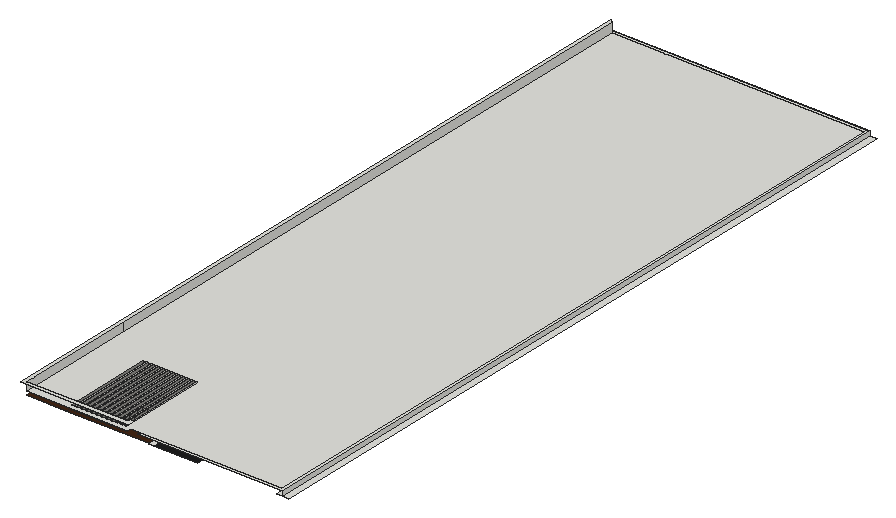
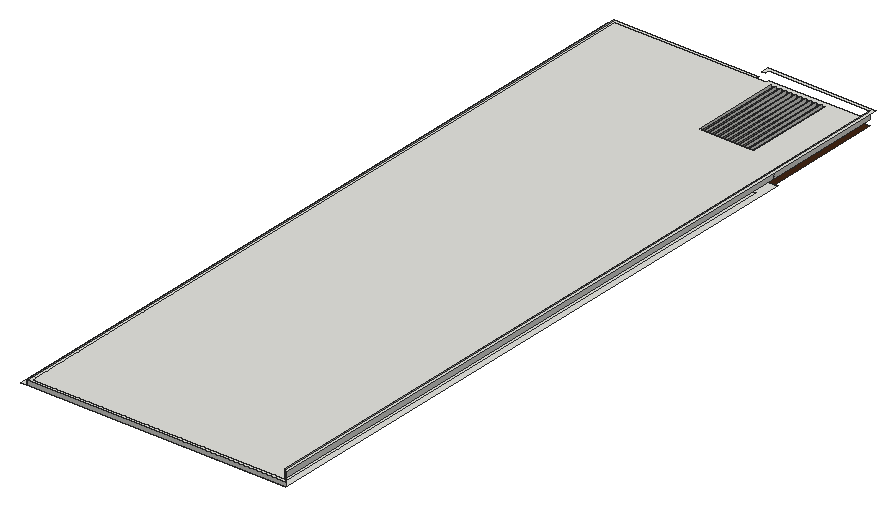
# SketchUp Ruby script. Lengths in inches.
U = 1.inch
M = Sketchup.active_model
def pt(a) = Geom::Point3d.new(a.map { |v| v * U })
def face(e, loops, mat)
  f = e.add_face(loops[0].map { |a| pt(a) })
  loops[1..].each { |l| e.add_face(l.map { |a| pt(a) }).erase! }
  f.material = f.back_material = mat if mat
  f
end
# faces: each face lists its corners as indices into pts; further lists are holes
def faces(e, pts, list, mat = nil) = list.each { |f| face(e, (f[0].is_a?(Array) ? f : [f]).map { |l| l.map { |i| pts[i] } }, mat) }
# xy, xz, yz: faces in a plane at the given z, y or x. An outline is a flat list of corners, or four numbers for a rectangle; further outlines are holes
def ring(l) = l.size == 4 ? [[l[0], l[1]], [l[2], l[1]], [l[2], l[3]], [l[0], l[3]]] : l.each_slice(2).to_a
def flat(e, list, mat, &to3) = list.each { |f| face(e, (f[0].is_a?(Array) ? f : [f]).map { |l| ring(l).map { |u, v| to3.(u, v) } }, mat) }
def xy(e, z, list, mat = nil) = flat(e, list, mat) { |x, y| [x, y, z] }
def xz(e, y, list, mat = nil) = flat(e, list, mat) { |x, z| [x, y, z] }
def yz(e, x, list, mat = nil) = flat(e, list, mat) { |y, z| [x, y, z] }
def lines(e, pts, list) = list.each { |a, b| e.add_line(pt(pts[a]), pt(pts[b])) }
# prism: a flat outline (further loops are holes) pulled along v
def prism(e, loops, v, mat = nil)
  f = face(e, loops, mat); d = Geom::Vector3d.new(v.map { |x| x * U })
  f.pushpull(f.normal.samedirection?(d) ? d.length : -d.length)
end
def box(e, o, s, mat = nil) = prism(e, [[o, [o[0] + s[0], o[1], o[2]], [o[0] + s[0], o[1] + s[1], o[2]], [o[0], o[1] + s[1], o[2]]]], [0, 0, s[2]], mat)
def at(x, y, z, deg = 0) = Geom::Transformation.translation(pt([x, y, z])) * Geom::Transformation.rotation(ORIGIN, Z_AXIS, deg.degrees)
def axes(o, x, y, z) = Geom::Transformation.new([*x, 0, *y, 0, *z, 0, *pt(o).to_a, 1])
def part(name) = M.definitions.add(name)
# library, detail: a bought-in or finely detailed component or shape, given as its bounding box
def library(name, o, s) = part(name).tap { |d| box(d.entities, o, s) }
def detail(e, o, s) = box(e.add_group.entities, o, s)
def put(e, d, t, mat = nil) = e.add_instance(d, t).tap { |i| i.material = mat if mat }
def group(e, t, mat = nil) = e.add_group.tap { |g| g.transformation = t; g.material = mat if mat }.entities
root = M.entities
M.materials.add("[Color M08]").color = [30, 30, 30]
M.materials.add("[Field Square Tile]").color = [211, 167, 108]
M.materials.add("[Granite Light Gray]").color = [149, 148, 144]
M.materials.add("[Wood Veneer 01]").color = [66, 38, 20]
xy(root,380.5,[[3312.79,511.08,3312.79,1825.82,2865.03,1825.82,2865.03,762.17,3081.03,762.17,3081.03,727.2,2855.22,727.2,2855.22,1835.625,3322.6,1835.625,3322.6,511.08],[3081.03,511.08,3089.95,589.83],[3322.6,511.08,3334.41,1835.625],[3081.03,589.83,3081.03,762.17,2865.03,762.17,2865.03,1825.82,3312.79,1825.82,3312.79,589.83,3266.02,589.83,3266.02,697.21,3170.71,697.21,3170.71,738.02,3089.95,738.02,3089.95,697.21,3081.33,697.21,3081.33,589.83],[3081.33,589.83,3089.95,697.21],
  [3170.71,589.83,3266.02,697.21],[3089.95,697.21,3170.71,738.02]])
xy(root,380.5,[[3089.95,511.08,3170.71,697.21]],"[Color M08]")
xy(root,380.5,[[[2860.05,512.27,2931.98,727.2],[2877.08,606.01,2878.6,606.38,2879.98,607.14,2881.11,608.22,2881.92,609.56,2882.35,611.0625,2882.39,612.63,2882.01,614.15,2881.26,615.52,2880.17,616.65,2878.83,617.46,2877.33,617.9,2875.76,617.93,2874.24,617.56,2872.87,616.81,2871.74,615.72,2870.93,614.38,2870.49,612.875,2870.46,611.3125,2870.83,609.79,2871.59,608.42,2872.67,607.29,2874.01,606.48,2875.52,606.04],[2877.08,554.26,2878.6,554.63,2879.98,555.39,2881.11,556.47,2881.92,557.81,2882.35,559.3125,2882.39,560.88,2882.01,562.4,2881.26,563.77,2880.17,564.9,2878.83,565.71,2877.33,566.15,2875.76,566.18,2874.24,565.81,2872.87,565.06,2871.74,563.97,2870.93,562.63,2870.49,561.125,2870.46,559.5625,2870.83,558.04,2871.59,556.67,2872.67,555.54,2874.01,554.73,2875.52,554.29],[2877.08,523.51,2878.6,523.88,2879.98,524.64,2881.11,525.72,2881.92,527.06,2882.35,528.5625,2882.39,530.13,2882.01,531.65,2881.26,533.02,2880.17,534.15,2878.83,534.96,2877.33,535.4,2875.76,535.43,2874.24,535.06,2872.87,534.31,2871.74,533.22,2870.93,531.88,2870.49,530.375,2870.46,528.8125,2870.83,527.29,2871.59,525.92,2872.67,524.79,2874.01,523.98,2875.52,523.54],[2877.08,666.01,2878.6,666.38,2879.98,667.14,2881.11,668.22,2881.92,669.56,2882.35,671.0625,2882.39,672.63,2882.01,674.15,2881.26,675.52,2880.17,676.65,2878.83,677.46,2877.33,677.9,2875.76,677.93,2874.24,677.56,2872.87,676.81,2871.74,675.72,2870.93,674.38,2870.49,672.875,2870.46,671.3125,2870.83,669.79,2871.59,668.42,2872.67,667.29,2874.01,666.48,2875.52,666.04],[2916.83,606.01,2918.35,606.38,2919.73,607.14,2920.86,608.22,2921.67,609.56,2922.1,611.0625,2922.14,612.63,2921.76,614.15,2921.01,615.52,2919.92,616.65,2918.58,617.46,2917.08,617.9,2915.51,617.93,2913.99,617.56,2912.62,616.81,2911.49,615.72,2910.68,614.38,2910.24,612.875,2910.21,611.3125,2910.58,609.79,2911.34,608.42,2912.42,607.29,2913.76,606.48,2915.27,606.04],[2916.83,554.26,2918.35,554.63,2919.73,555.39,2920.86,556.47,2921.67,557.81,2922.1,559.3125,2922.14,560.88,2921.76,562.4,2921.01,563.77,2919.92,564.9,2918.58,565.71,2917.08,566.15,2915.51,566.18,2913.99,565.81,2912.62,565.06,2911.49,563.97,2910.68,562.63,2910.24,561.125,2910.21,559.5625,2910.58,558.04,2911.34,556.67,2912.42,555.54,2913.76,554.73,2915.27,554.29],[2916.83,523.51,2918.35,523.88,2919.73,524.64,2920.86,525.72,2921.67,527.06,2922.1,528.5625,2922.14,530.13,2921.76,531.65,2921.01,533.02,2919.92,534.15,2918.58,534.96,2917.08,535.4,2915.51,535.43,2913.99,535.06,2912.62,534.31,2911.49,533.22,2910.68,531.88,2910.24,530.375,2910.21,528.8125,2910.58,527.29,2911.34,525.92,2912.42,524.79,2913.76,523.98,2915.27,523.54],[2916.83,666.01,2918.35,666.38,2919.73,667.14,2920.86,668.22,2921.67,669.56,2922.1,671.0625,2922.14,672.63,2921.76,674.15,2921.01,675.52,2919.92,676.65,2918.58,677.46,2917.08,677.9,2915.51,677.93,2913.99,677.56,2912.62,676.81,2911.49,675.72,2910.68,674.38,2910.24,672.875,2910.21,671.3125,2910.58,669.79,2911.34,668.42,2912.42,667.29,2913.76,666.48,2915.27,666.04]],[[2931.98,512.27,3081.03,727.2],[3027.43,519.43,3033.68,680.49],[3018.31,519.43,3024.56,680.49],[3009.18,519.43,3015.43,680.49],[3000.06,519.43,3006.31,680.49],[2990.93,519.43,2997.18,680.49],[2981.81,519.43,2988.06,680.49],[2972.68,519.43,2978.93,680.49],[2963.56,519.43,2969.81,680.49],[2954.43,519.43,2960.68,680.49],[2945.31,519.43,2951.56,680.49],[2936.18,519.43,2942.43,680.49]]],"[Wood Veneer 01]")
xy(root,381.875,[[2877.08,554.26,2875.52,554.29,2874.01,554.73,2872.67,555.54,2871.59,556.67,2870.83,558.04,2870.46,559.5625,2870.49,561.125,2870.93,562.63,2871.74,563.97,2872.87,565.06,2874.24,565.81,2875.76,566.18,2877.33,566.15,2878.83,565.71,2880.17,564.9,2881.26,563.77,2882.01,562.4,2882.39,560.88,2882.35,559.3125,2881.92,557.81,2881.11,556.47,2879.98,555.39,2878.6,554.63],[2916.83,554.26,2915.27,554.29,2913.76,554.73,2912.42,555.54,2911.34,556.67,2910.58,558.04,2910.21,559.5625,2910.24,561.125,2910.68,562.63,2911.49,563.97,2912.62,565.06,2913.99,565.81,2915.51,566.18,2917.08,566.15,2918.58,565.71,2919.92,564.9,2921.01,563.77,2921.76,562.4,2922.14,560.88,2922.1,559.3125,2921.67,557.81,2920.86,556.47,2919.73,555.39,2918.35,554.63],[2877.08,606.01,2875.52,606.04,2874.01,606.48,2872.67,607.29,2871.59,608.42,2870.83,609.79,2870.46,611.3125,2870.49,612.875,2870.93,614.38,2871.74,615.72,2872.87,616.81,2874.24,617.56,2875.76,617.93,2877.33,617.9,2878.83,617.46,2880.17,616.65,2881.26,615.52,2882.01,614.15,2882.39,612.63,2882.35,611.0625,2881.92,609.56,2881.11,608.22,2879.98,607.14,2878.6,606.38],[2916.83,606.01,2915.27,606.04,2913.76,606.48,2912.42,607.29,2911.34,608.42,2910.58,609.79,2910.21,611.3125,2910.24,612.875,2910.68,614.38,2911.49,615.72,2912.62,616.81,2913.99,617.56,2915.51,617.93,2917.08,617.9,2918.58,617.46,2919.92,616.65,2921.01,615.52,2921.76,614.15,2922.14,612.63,2922.1,611.0625,2921.67,609.56,2920.86,608.22,2919.73,607.14,2918.35,606.38],[2877.08,666.01,2875.52,666.04,2874.01,666.48,2872.67,667.29,2871.59,668.42,2870.83,669.79,2870.46,671.3125,2870.49,672.875,2870.93,674.38,2871.74,675.72,2872.87,676.81,2874.24,677.56,2875.76,677.93,2877.33,677.9,2878.83,677.46,2880.17,676.65,2881.26,675.52,2882.01,674.15,2882.39,672.63,2882.35,671.0625,2881.92,669.56,2881.11,668.22,2879.98,667.14,2878.6,666.38],
  [2916.83,666.01,2915.27,666.04,2913.76,666.48,2912.42,667.29,2911.34,668.42,2910.58,669.79,2910.21,671.3125,2910.24,672.875,2910.68,674.38,2911.49,675.72,2912.62,676.81,2913.99,677.56,2915.51,677.93,2917.08,677.9,2918.58,677.46,2919.92,676.65,2921.01,675.52,2921.76,674.15,2922.14,672.63,2922.1,671.0625,2921.67,669.56,2920.86,668.22,2919.73,667.14,2918.35,666.38]],"[Field Square Tile]")
xy(root,388.625,[[[2861.56,510.87,3044.88,510.87,3044.88,517.43,3316.25,517.43,3316.25,1829.28,2861.56,1829.28],[2936.18,519.43,2942.43,680.49],[2945.31,519.43,2951.56,680.49],[2954.43,519.43,2960.68,680.49],[2963.56,519.43,2969.81,680.49],[2972.68,519.43,2978.93,680.49],[2981.81,519.43,2988.06,680.49],[2990.93,519.43,2997.18,680.49],[3000.06,519.43,3006.31,680.49],[3009.18,519.43,3015.43,680.49],[3018.31,519.43,3024.56,680.49],[3027.43,519.43,3033.68,680.49]],[3061.9375,511.08,3322.6,511.08,3322.6,1835.625,2855.22,1835.625,2861.56,1829.28,3316.25,1829.28,3316.25,517.43,3061.9375,517.43]])
xy(root,403.8125,[[2855.22,504.52,3051.23,504.52,3051.23,517.43,3044.88,517.43,3044.88,510.87,2861.56,510.87,2861.56,1829.28,2855.22,1835.625]])
xz(root,680.49,[[2936.18,380.5,2942.43,388.625],[2945.31,380.5,2951.56,388.625],[2954.43,380.5,2960.68,388.625],[2963.56,380.5,2969.81,388.625],[2972.68,380.5,2978.93,388.625],
  [2981.81,380.5,2988.06,388.625],[2990.93,380.5,2997.18,388.625],[3000.06,380.5,3006.31,388.625],[3009.18,380.5,3015.43,388.625],[3018.31,380.5,3024.56,388.625],
  [3027.43,380.5,3033.68,388.625]],"[Granite Light Gray]")
xz(root,1835.625,[[2855.22,380.5,3322.6,388.625]])
yz(root,2861.56,[[510.87,388.625,727.2,403.8125],[727.2,388.625,1829.28,403.8125]])
yz(root,2936.18,[[519.43,380.5,680.49,388.625]],"[Granite Light Gray]")
yz(root,2942.43,[[519.43,380.5,680.49,388.625]])
yz(root,2945.31,[[519.43,380.5,680.49,388.625]],"[Granite Light Gray]")
yz(root,2951.56,[[519.43,380.5,680.49,388.625]])
yz(root,2954.43,[[519.43,380.5,680.49,388.625]],"[Granite Light Gray]")
yz(root,2960.68,[[519.43,380.5,680.49,388.625]])
yz(root,2963.56,[[519.43,380.5,680.49,388.625]],"[Granite Light Gray]")
yz(root,2969.81,[[519.43,380.5,680.49,388.625]])
yz(root,2972.68,[[519.43,380.5,680.49,388.625]],"[Granite Light Gray]")
yz(root,2978.93,[[519.43,380.5,680.49,388.625]])
yz(root,2981.81,[[519.43,380.5,680.49,388.625]],"[Granite Light Gray]")
yz(root,2988.06,[[519.43,380.5,680.49,388.625]])
yz(root,2990.93,[[519.43,380.5,680.49,388.625]],"[Granite Light Gray]")
yz(root,2997.18,[[519.43,380.5,680.49,388.625]])
yz(root,3000.06,[[519.43,380.5,680.49,388.625]],"[Granite Light Gray]")
yz(root,3006.31,[[519.43,380.5,680.49,388.625]])
yz(root,3009.18,[[519.43,380.5,680.49,388.625]],"[Granite Light Gray]")
yz(root,3015.43,[[519.43,380.5,680.49,388.625]])
yz(root,3018.31,[[519.43,380.5,680.49,388.625]],"[Granite Light Gray]")
yz(root,3024.56,[[519.43,380.5,680.49,388.625]])
yz(root,3027.43,[[519.43,380.5,680.49,388.625]],"[Granite Light Gray]")
yz(root,3033.68,[[519.43,380.5,680.49,388.625]])
yz(root,3322.6,[[511.08,380.5,1835.625,388.625]])
p = [[2875.76,535.43,380.5],[2877.33,535.4,380.5],[2877.33,535.4,381.875],[2875.76,535.43,381.875],[2915.51,535.43,380.5],[2917.08,535.4,380.5],
  [2917.08,535.4,381.875],[2915.51,535.43,381.875],[2875.52,554.29,380.5],[2874.01,554.73,380.5],[2874.01,554.73,381.875],[2875.52,554.29,381.875],
  [2877.08,554.26,380.5],[2877.08,554.26,381.875],[2878.6,554.63,380.5],[2878.6,554.63,381.875],[2915.27,554.29,380.5],[2913.76,554.73,380.5],
  [2913.76,554.73,381.875],[2915.27,554.29,381.875],[2916.83,554.26,380.5],[2916.83,554.26,381.875],[2918.35,554.63,380.5],[2918.35,554.63,381.875],
  [2879.98,555.39,380.5],[2879.98,555.39,381.875],[2919.73,555.39,380.5],[2919.73,555.39,381.875],[2872.67,555.54,380.5],[2872.67,555.54,381.875],
  [2912.42,555.54,380.5],[2912.42,555.54,381.875],[2881.11,556.47,380.5],[2881.11,556.47,381.875],[2920.86,556.47,380.5],[2920.86,556.47,381.875],
  [2871.59,556.67,380.5],[2871.59,556.67,381.875],[2911.34,556.67,380.5],[2911.34,556.67,381.875],[2881.92,557.81,380.5],[2881.92,557.81,381.875],
  [2921.67,557.81,380.5],[2921.67,557.81,381.875],[2870.83,558.04,380.5],[2870.83,558.04,381.875],[2910.58,558.04,380.5],[2910.58,558.04,381.875],
  [2882.35,559.3125,380.5],[2882.35,559.3125,381.875],[2922.1,559.3125,380.5],[2922.1,559.3125,381.875],[2870.46,559.5625,380.5],[2870.46,559.5625,381.875],
  [2910.21,559.5625,380.5],[2910.21,559.5625,381.875],[2882.39,560.88,380.5],[2882.39,560.88,381.875],[2922.14,560.88,380.5],[2922.14,560.88,381.875],
  [2870.49,561.125,380.5],[2870.49,561.125,381.875],[2910.24,561.125,380.5],[2910.24,561.125,381.875],[2882.01,562.4,380.5],[2882.01,562.4,381.875],
  [2921.76,562.4,380.5],[2921.76,562.4,381.875],[2870.93,562.63,380.5],[2870.93,562.63,381.875],[2910.68,562.63,380.5],[2910.68,562.63,381.875],
  [2881.26,563.77,380.5],[2881.26,563.77,381.875],[2921.01,563.77,380.5],[2921.01,563.77,381.875],[2871.74,563.97,380.5],[2871.74,563.97,381.875],
  [2911.49,563.97,380.5],[2911.49,563.97,381.875],[2880.17,564.9,380.5],[2880.17,564.9,381.875],[2919.92,564.9,380.5],[2919.92,564.9,381.875],
  [2872.87,565.06,380.5],[2872.87,565.06,381.875],[2912.62,565.06,380.5],[2912.62,565.06,381.875],[2878.83,565.71,380.5],[2878.83,565.71,381.875],
  [2918.58,565.71,380.5],[2918.58,565.71,381.875],[2874.24,565.81,380.5],[2874.24,565.81,381.875],[2913.99,565.81,380.5],[2913.99,565.81,381.875],
  [2877.33,566.15,380.5],[2877.33,566.15,381.875],[2917.08,566.15,380.5],[2917.08,566.15,381.875],[2875.76,566.18,380.5],[2875.76,566.18,381.875],
  [2915.51,566.18,380.5],[2915.51,566.18,381.875],[2875.52,606.04,380.5],[2874.01,606.48,380.5],[2874.01,606.48,381.875],[2875.52,606.04,381.875],
  [2877.08,606.01,380.5],[2877.08,606.01,381.875],[2878.6,606.38,380.5],[2878.6,606.38,381.875],[2915.27,606.04,380.5],[2913.76,606.48,380.5],
  [2913.76,606.48,381.875],[2915.27,606.04,381.875],[2916.83,606.01,380.5],[2916.83,606.01,381.875],[2918.35,606.38,380.5],[2918.35,606.38,381.875],
  [2879.98,607.14,380.5],[2879.98,607.14,381.875],[2919.73,607.14,380.5],[2919.73,607.14,381.875],[2872.67,607.29,380.5],[2872.67,607.29,381.875],
  [2912.42,607.29,380.5],[2912.42,607.29,381.875],[2881.11,608.22,380.5],[2881.11,608.22,381.875],[2920.86,608.22,380.5],[2920.86,608.22,381.875],
  [2871.59,608.42,380.5],[2871.59,608.42,381.875],[2911.34,608.42,380.5],[2911.34,608.42,381.875],[2881.92,609.56,380.5],[2881.92,609.56,381.875],
  [2921.67,609.56,380.5],[2921.67,609.56,381.875],[2870.83,609.79,380.5],[2870.83,609.79,381.875],[2910.58,609.79,380.5],[2910.58,609.79,381.875],
  [2882.35,611.0625,380.5],[2882.35,611.0625,381.875],[2922.1,611.0625,380.5],[2922.1,611.0625,381.875],[2870.46,611.3125,380.5],[2870.46,611.3125,381.875],
  [2910.21,611.3125,380.5],[2910.21,611.3125,381.875],[2882.39,612.63,380.5],[2882.39,612.63,381.875],[2922.14,612.63,380.5],[2922.14,612.63,381.875],
  [2870.49,612.875,380.5],[2870.49,612.875,381.875],[2910.24,612.875,380.5],[2910.24,612.875,381.875],[2882.01,614.15,380.5],[2882.01,614.15,381.875],
  [2921.76,614.15,380.5],[2921.76,614.15,381.875],[2870.93,614.38,380.5],[2870.93,614.38,381.875],[2910.68,614.38,380.5],[2910.68,614.38,381.875],
  [2881.26,615.52,380.5],[2881.26,615.52,381.875],[2921.01,615.52,380.5],[2921.01,615.52,381.875],[2871.74,615.72,380.5],[2871.74,615.72,381.875],
  [2911.49,615.72,380.5],[2911.49,615.72,381.875],[2880.17,616.65,380.5],[2880.17,616.65,381.875],[2919.92,616.65,380.5],[2919.92,616.65,381.875],
  [2872.87,616.81,380.5],[2872.87,616.81,381.875],[2912.62,616.81,380.5],[2912.62,616.81,381.875],[2878.83,617.46,380.5],[2878.83,617.46,381.875],
  [2918.58,617.46,380.5],[2918.58,617.46,381.875],[2874.24,617.56,380.5],[2874.24,617.56,381.875],[2913.99,617.56,380.5],[2913.99,617.56,381.875],
  [2877.33,617.9,380.5],[2877.33,617.9,381.875],[2917.08,617.9,380.5],[2917.08,617.9,381.875],[2875.76,617.93,380.5],[2875.76,617.93,381.875],
  [2915.51,617.93,380.5],[2915.51,617.93,381.875],[2875.52,666.04,380.5],[2874.01,666.48,380.5],[2874.01,666.48,381.875],[2875.52,666.04,381.875],
  [2877.08,666.01,380.5],[2877.08,666.01,381.875],[2878.6,666.38,380.5],[2878.6,666.38,381.875],[2915.27,666.04,380.5],[2913.76,666.48,380.5],
  [2913.76,666.48,381.875],[2915.27,666.04,381.875],[2916.83,666.01,380.5],[2916.83,666.01,381.875],[2918.35,666.38,380.5],[2918.35,666.38,381.875],
  [2879.98,667.14,380.5],[2879.98,667.14,381.875],[2919.73,667.14,380.5],[2919.73,667.14,381.875],[2872.67,667.29,380.5],[2872.67,667.29,381.875],
  [2912.42,667.29,380.5],[2912.42,667.29,381.875],[2881.11,668.22,380.5],[2881.11,668.22,381.875],[2920.86,668.22,380.5],[2920.86,668.22,381.875],
  [2871.59,668.42,380.5],[2871.59,668.42,381.875],[2911.34,668.42,380.5],[2911.34,668.42,381.875],[2881.92,669.56,380.5],[2881.92,669.56,381.875],
  [2921.67,669.56,380.5],[2921.67,669.56,381.875],[2870.83,669.79,380.5],[2870.83,669.79,381.875],[2910.58,669.79,380.5],[2910.58,669.79,381.875],
  [2882.35,671.0625,380.5],[2882.35,671.0625,381.875],[2922.1,671.0625,380.5],[2922.1,671.0625,381.875],[2870.46,671.3125,380.5],[2870.46,671.3125,381.875],
  [2910.21,671.3125,380.5],[2910.21,671.3125,381.875],[2882.39,672.63,380.5],[2882.39,672.63,381.875],[2922.14,672.63,380.5],[2922.14,672.63,381.875],
  [2870.49,672.875,380.5],[2870.49,672.875,381.875],[2910.24,672.875,380.5],[2910.24,672.875,381.875],[2882.01,674.15,380.5],[2882.01,674.15,381.875],
  [2921.76,674.15,380.5],[2921.76,674.15,381.875],[2870.93,674.38,380.5],[2870.93,674.38,381.875],[2910.68,674.38,380.5],[2910.68,674.38,381.875],
  [2881.26,675.52,380.5],[2881.26,675.52,381.875],[2921.01,675.52,380.5],[2921.01,675.52,381.875],[2871.74,675.72,380.5],[2871.74,675.72,381.875],
  [2911.49,675.72,380.5],[2911.49,675.72,381.875],[2880.17,676.65,380.5],[2880.17,676.65,381.875],[2919.92,676.65,380.5],[2919.92,676.65,381.875],
  [2872.87,676.81,380.5],[2872.87,676.81,381.875],[2912.62,676.81,380.5],[2912.62,676.81,381.875],[2878.83,677.46,380.5],[2878.83,677.46,381.875],
  [2918.58,677.46,380.5],[2918.58,677.46,381.875],[2874.24,677.56,380.5],[2874.24,677.56,381.875],[2913.99,677.56,380.5],[2913.99,677.56,381.875],
  [2877.33,677.9,380.5],[2877.33,677.9,381.875],[2917.08,677.9,380.5],[2917.08,677.9,381.875],[2875.76,677.93,380.5],[2875.76,677.93,381.875],
  [2915.51,677.93,380.5],[2915.51,677.93,381.875],[2861.56,1829.28,388.625],[2855.22,1835.625,388.625],[2855.22,1835.625,403.8125],[2861.56,1829.28,403.8125]]
faces(root,p,[[0,1,2,3],[4,5,6,7],[8,9,10,11],[12,8,11,13],[14,12,13,15],[16,17,18,19],[20,16,19,21],[22,20,21,23],
  [24,14,15,25],[26,22,23,27],[9,28,29,10],[17,30,31,18],[32,24,25,33],[34,26,27,35],[28,36,37,29],[30,38,39,31],
  [40,32,33,41],[42,34,35,43],[36,44,45,37],[38,46,47,39],[48,40,41,49],[50,42,43,51],[44,52,53,45],[46,54,55,47],
  [56,48,49,57],[58,50,51,59],[52,60,61,53],[54,62,63,55],[64,56,57,65],[66,58,59,67],[60,68,69,61],[62,70,71,63],
  [72,64,65,73],[74,66,67,75],[68,76,77,69],[70,78,79,71],[80,72,73,81],[82,74,75,83],[76,84,85,77],[78,86,87,79],
  [88,80,81,89],[90,82,83,91],[84,92,93,85],[86,94,95,87],[96,88,89,97],[98,90,91,99],[92,100,101,93],[94,102,103,95],
  [100,96,97,101],[102,98,99,103],[104,105,106,107],[108,104,107,109],[110,108,109,111],[112,113,114,115],[116,112,115,117],[118,116,117,119],
  [120,110,111,121],[122,118,119,123],[105,124,125,106],[113,126,127,114],[128,120,121,129],[130,122,123,131],[124,132,133,125],[126,134,135,127],
  [136,128,129,137],[138,130,131,139],[132,140,141,133],[134,142,143,135],[144,136,137,145],[146,138,139,147],[140,148,149,141],[142,150,151,143],
  [152,144,145,153],[154,146,147,155],[148,156,157,149],[150,158,159,151],[160,152,153,161],[162,154,155,163],[156,164,165,157],[158,166,167,159],
  [168,160,161,169],[170,162,163,171],[164,172,173,165],[166,174,175,167],[176,168,169,177],[178,170,171,179],[172,180,181,173],[174,182,183,175],
  [184,176,177,185],[186,178,179,187],[180,188,189,181],[182,190,191,183],[192,184,185,193],[194,186,187,195],[188,196,197,189],[190,198,199,191],
  [196,192,193,197],[198,194,195,199],[200,201,202,203],[204,200,203,205],[206,204,205,207],[208,209,210,211],[212,208,211,213],[214,212,213,215],
  [216,206,207,217],[218,214,215,219],[201,220,221,202],[209,222,223,210],[224,216,217,225],[226,218,219,227],[220,228,229,221],[222,230,231,223],
  [232,224,225,233],[234,226,227,235],[228,236,237,229],[230,238,239,231],[240,232,233,241],[242,234,235,243],[236,244,245,237],[238,246,247,239],
  [248,240,241,249],[250,242,243,251],[244,252,253,245],[246,254,255,247],[256,248,249,257],[258,250,251,259],[252,260,261,253],[254,262,263,255],
  [264,256,257,265],[266,258,259,267],[260,268,269,261],[262,270,271,263],[272,264,265,273],[274,266,267,275],[268,276,277,269],[270,278,279,271],
  [280,272,273,281],[282,274,275,283],[276,284,285,277],[278,286,287,279],[288,280,281,289],[290,282,283,291],[284,292,293,285],[286,294,295,287],
  [292,288,289,293],[294,290,291,295]],"[Field Square Tile]")
faces(root,p,[[296,297,298,299]])
